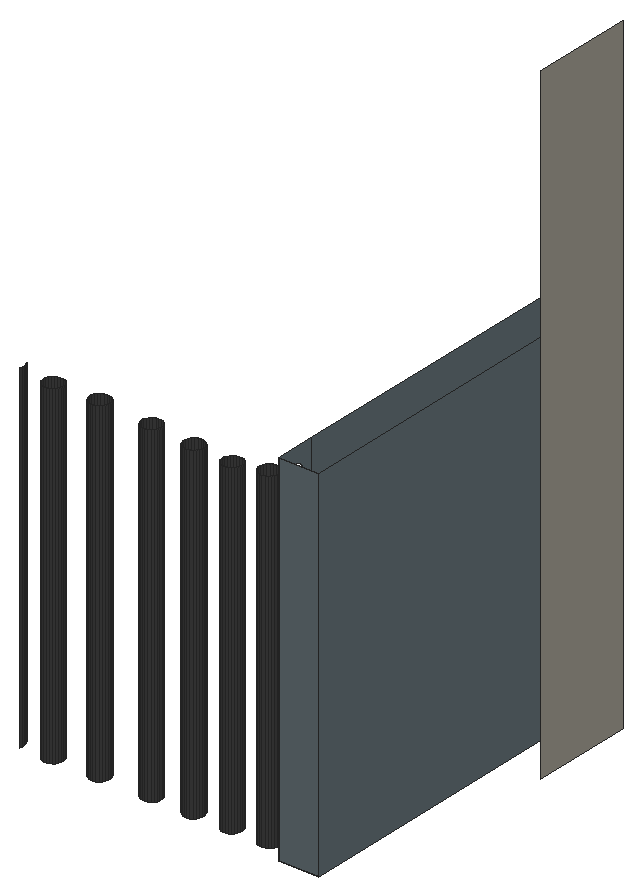
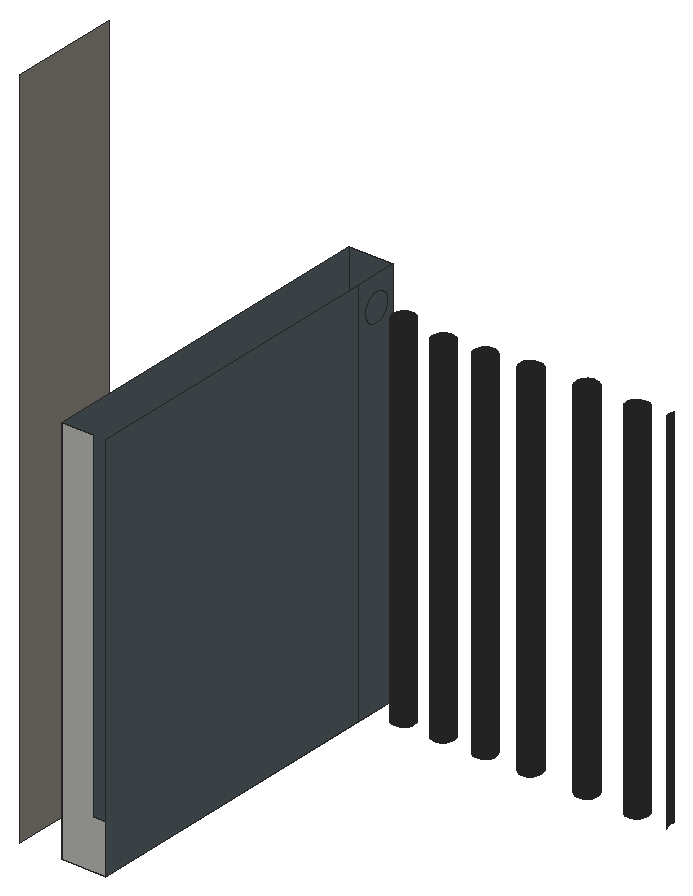
# SketchUp Ruby script. Lengths in inches.
U = 1.inch
M = Sketchup.active_model
def pt(a) = Geom::Point3d.new(a.map { |v| v * U })
def face(e, loops, mat)
  f = e.add_face(loops[0].map { |a| pt(a) })
  loops[1..].each { |l| e.add_face(l.map { |a| pt(a) }).erase! }
  f.material = f.back_material = mat if mat
  f
end
# faces: each face lists its corners as indices into pts; further lists are holes
def faces(e, pts, list, mat = nil) = list.each { |f| face(e, (f[0].is_a?(Array) ? f : [f]).map { |l| l.map { |i| pts[i] } }, mat) }
# xy, xz, yz: faces in a plane at the given z, y or x. An outline is a flat list of corners, or four numbers for a rectangle; further outlines are holes
def ring(l) = l.size == 4 ? [[l[0], l[1]], [l[2], l[1]], [l[2], l[3]], [l[0], l[3]]] : l.each_slice(2).to_a
def flat(e, list, mat, &to3) = list.each { |f| face(e, (f[0].is_a?(Array) ? f : [f]).map { |l| ring(l).map { |u, v| to3.(u, v) } }, mat) }
def xy(e, z, list, mat = nil) = flat(e, list, mat) { |x, y| [x, y, z] }
def xz(e, y, list, mat = nil) = flat(e, list, mat) { |x, z| [x, y, z] }
def yz(e, x, list, mat = nil) = flat(e, list, mat) { |y, z| [x, y, z] }
def lines(e, pts, list) = list.each { |a, b| e.add_line(pt(pts[a]), pt(pts[b])) }
# prism: a flat outline (further loops are holes) pulled along v
def prism(e, loops, v, mat = nil)
  f = face(e, loops, mat); d = Geom::Vector3d.new(v.map { |x| x * U })
  f.pushpull(f.normal.samedirection?(d) ? d.length : -d.length)
end
def box(e, o, s, mat = nil) = prism(e, [[o, [o[0] + s[0], o[1], o[2]], [o[0] + s[0], o[1] + s[1], o[2]], [o[0], o[1] + s[1], o[2]]]], [0, 0, s[2]], mat)
def at(x, y, z, deg = 0) = Geom::Transformation.translation(pt([x, y, z])) * Geom::Transformation.rotation(ORIGIN, Z_AXIS, deg.degrees)
def axes(o, x, y, z) = Geom::Transformation.new([*x, 0, *y, 0, *z, 0, *pt(o).to_a, 1])
def part(name) = M.definitions.add(name)
# library, detail: a bought-in or finely detailed component or shape, given as its bounding box
def library(name, o, s) = part(name).tap { |d| box(d.entities, o, s) }
def detail(e, o, s) = box(e.add_group.entities, o, s)
def put(e, d, t, mat = nil) = e.add_instance(d, t).tap { |i| i.material = mat if mat }
def group(e, t, mat = nil) = e.add_group.tap { |g| g.transformation = t; g.material = mat if mat }.entities
root = M.entities
M.materials.add("[Color M07]").color = [58, 58, 58]
M.materials.add("[Formica Graystone]").color = [149, 146, 135]
M.materials.add("[Formica Speckled Grey]").color = [94, 105, 111]
xy(root,334.79,[[295.92,120.91,298.73,144.04],[279.04,121.51,278.87,121.56,278.71,121.65,278.59,121.78,278.5,121.93,278.46,122.11,278.46,122.28,278.51,122.46,278.6,122.61,278.73,122.74,278.88,122.83,279.06,122.87,279.23,122.87,279.41,122.82,279.5625,122.73,279.6875,122.6,279.78,122.45,279.82,122.27,279.82,122.09,279.77,121.92,279.68,121.76,279.55,121.64,279.4,121.55,279.22,121.51],[282.29,121.51,282.12,121.56,281.96,121.65,281.84,121.78,281.75,121.93,281.71,122.11,281.71,122.28,281.76,122.46,281.85,122.61,281.98,122.74,282.13,122.83,282.31,122.87,282.48,122.87,282.66,122.82,282.8125,122.73,282.9375,122.6,283.03,122.45,283.07,122.27,283.07,122.09,283.02,121.92,282.93,121.76,282.8,121.64,282.65,121.55,282.47,121.51],[285.92,121.51,285.74,121.56,285.59,121.65,285.46,121.78,285.375,121.93,285.33,122.11,285.33,122.28,285.38,122.46,285.47,122.61,285.6,122.74,285.76,122.83,285.93,122.87,286.11,122.87,286.28,122.82,286.4375,122.73,286.5625,122.6,286.65,122.45,286.7,122.27,286.69,122.09,286.65,121.92,286.55,121.76,286.43,121.64,286.27,121.55,286.1,121.51],[288.85,121.51,288.68,121.56,288.53,121.65,288.4,121.78,288.3125,121.93,288.27,122.11,288.27,122.28,288.32,122.46,288.41,122.61,288.54,122.74,288.69,122.83,288.87,122.87,289.05,122.87,289.22,122.82,289.375,122.73,289.5,122.6,289.59,122.45,289.63,122.27,289.63,122.09,289.58,121.92,289.49,121.76,289.36,121.64,289.21,121.55,289.03,121.51],
  [291.54,121.51,291.37,121.56,291.21,121.65,291.09,121.78,291,121.93,290.96,122.11,290.96,122.28,291.01,122.46,291.1,122.61,291.23,122.74,291.38,122.83,291.56,122.87,291.73,122.87,291.91,122.82,292.0625,122.73,292.1875,122.6,292.28,122.45,292.32,122.27,292.32,122.09,292.27,121.92,292.18,121.76,292.05,121.64,291.9,121.55,291.72,121.51],[294.1,121.51,293.93,121.56,293.78,121.65,293.65,121.78,293.5625,121.93,293.52,122.11,293.52,122.28,293.57,122.46,293.66,122.61,293.79,122.74,293.94,122.83,294.12,122.87,294.3,122.87,294.47,122.82,294.625,122.73,294.75,122.6,294.84,122.45,294.88,122.27,294.88,122.09,294.83,121.92,294.74,121.76,294.61,121.64,294.46,121.55,294.28,121.51]])
xz(root,120.91,[[295.92,334.79,298.73,359.98]],"[Formica Speckled Grey]")
xz(root,121.51,[[279.04,334.79,279.22,358.23],[282.29,334.79,282.47,358.31],[285.92,334.79,286.1,358.07],[288.85,334.79,289.03,357.82],[291.54,334.79,291.72,357.67],
  [294.1,334.79,294.28,358.04]],"[Color M07]")
xz(root,122.87,[[279.06,334.79,279.23,358.23],[282.31,334.79,282.48,358.31],[285.93,334.79,286.11,358.07],[288.87,334.79,289.05,357.82],[291.56,334.79,291.73,357.67],
  [294.12,334.79,294.3,358.04]],"[Color M07]")
xz(root,144.04,[[295.92,334.79,298.73,334.79,298.73,359.98,296.73,359.98,296.73,337.93,295.92,337.93]])
yz(root,277.07,[[122.09,334.79,122.27,358.53]],"[Color M07]")
yz(root,278.46,[[122.11,334.79,122.28,358.23]],"[Color M07]")
yz(root,279.82,[[122.09,334.79,122.27,358.23]],"[Color M07]")
yz(root,281.71,[[122.11,334.79,122.28,358.31]],"[Color M07]")
yz(root,283.07,[[122.09,334.79,122.27,358.31]],"[Color M07]")
yz(root,285.33,[[122.11,334.79,122.28,358.07]],"[Color M07]")
yz(root,288.27,[[122.11,334.79,122.28,357.82]],"[Color M07]")
yz(root,289.63,[[122.09,334.79,122.27,357.82]],"[Color M07]")
yz(root,290.96,[[122.11,334.79,122.28,357.67]],"[Color M07]")
yz(root,292.32,[[122.09,334.79,122.27,357.67]],"[Color M07]")
yz(root,293.52,[[122.11,334.79,122.28,358.04]],"[Color M07]")
yz(root,294.88,[[122.09,334.79,122.27,358.04]],"[Color M07]")
yz(root,295.92,[[[120.91,334.79,123.73,359.98],[122.22,357.13,122.46,357.16,122.6875,357.25,122.88,357.4,123.03,357.6,123.125,357.82,123.16,358.07,123.125,358.31,123.03,358.53,122.88,358.73,122.6875,358.88,122.46,358.97,122.22,359,121.97,358.97,121.75,358.88,121.55,358.73,121.41,358.53,121.3125,358.31,121.28,358.07,121.3125,357.82,121.41,357.6,121.55,357.4,121.75,357.25,121.97,357.16]],[123.73,334.79,144.04,359.98]],"[Formica Speckled Grey]")
yz(root,298.73,[[120.91,334.79,144.04,359.98]],"[Formica Speckled Grey]")
yz(root,301.43,[[136.91,334.79,144.04,379.13]],"[Formica Graystone]")
p = [[278.87,121.56,334.79],[279.04,121.51,334.79],[279.04,121.51,358.23],[278.87,121.56,358.23],[278.87,121.56,357.4],[279.22,121.51,334.79],
  [279.4,121.55,334.79],[279.4,121.55,358.23],[279.22,121.51,358.23],[282.12,121.56,334.79],[282.29,121.51,334.79],[282.29,121.51,358.31],
  [282.12,121.56,358.31],[282.12,121.56,357.4],[282.47,121.51,334.79],[282.65,121.55,334.79],[282.65,121.55,358.31],[282.47,121.51,358.31],
  [285.74,121.56,334.79],[285.92,121.51,334.79],[285.92,121.51,358.07],[285.74,121.56,358.07],[285.74,121.56,357.4],[286.1,121.51,334.79],
  [286.27,121.55,334.79],[286.27,121.55,358.07],[286.1,121.51,358.07],[288.68,121.56,334.79],[288.85,121.51,334.79],[288.85,121.51,357.82],
  [288.68,121.56,357.82],[288.68,121.56,357.4],[289.03,121.51,334.79],[289.21,121.55,334.79],[289.21,121.55,357.82],[289.03,121.51,357.82],
  [291.37,121.56,334.79],[291.54,121.51,334.79],[291.54,121.51,357.67],[291.37,121.56,357.67],[291.37,121.56,357.4],[291.72,121.51,334.79],
  [291.9,121.55,334.79],[291.9,121.55,357.67],[291.72,121.51,357.67],[293.93,121.56,334.79],[294.1,121.51,334.79],[294.1,121.51,358.04],
  [293.93,121.56,358.04],[293.93,121.56,357.4],[294.28,121.51,334.79],[294.46,121.55,334.79],[294.46,121.55,358.04],[294.28,121.51,358.04],
  [278.59,121.78,334.79],[278.71,121.65,334.79],[278.71,121.65,358.23],[278.59,121.78,358.23],[279.55,121.64,334.79],[279.55,121.64,358.23],
  [279.68,121.76,334.79],[279.68,121.76,358.23],[281.84,121.78,334.79],[281.96,121.65,334.79],[281.96,121.65,358.31],[281.84,121.78,358.31],
  [282.8,121.64,334.79],[282.8,121.64,358.31],[282.93,121.76,334.79],[282.93,121.76,358.31],[285.46,121.78,334.79],[285.59,121.65,334.79],
  [285.59,121.65,358.07],[285.46,121.78,358.07],[286.43,121.64,334.79],[286.43,121.64,358.07],[286.55,121.76,334.79],[286.55,121.76,358.07],
  [288.4,121.78,334.79],[288.53,121.65,334.79],[288.53,121.65,357.82],[288.4,121.78,357.82],[289.36,121.64,334.79],[289.36,121.64,357.82],
  [289.49,121.76,334.79],[289.49,121.76,357.82],[291.09,121.78,334.79],[291.21,121.65,334.79],[291.21,121.65,357.67],[291.09,121.78,357.67],
  [292.05,121.64,334.79],[292.05,121.64,357.67],[292.18,121.76,334.79],[292.18,121.76,357.67],[293.65,121.78,334.79],[293.78,121.65,334.79],
  [293.78,121.65,358.04],[293.65,121.78,358.04],[294.61,121.64,334.79],[294.61,121.64,358.04],[294.74,121.76,334.79],[294.74,121.76,358.04],
  [278.5,121.93,334.79],[278.5,121.93,358.23],[279.77,121.92,334.79],[279.77,121.92,358.23],[281.75,121.93,334.79],[281.75,121.93,358.31],
  [283.02,121.92,334.79],[283.02,121.92,358.31],[285.375,121.93,334.79],[285.375,121.93,358.07],[286.65,121.92,334.79],[286.65,121.92,358.07],
  [288.3125,121.93,334.79],[288.3125,121.93,357.82],[289.58,121.92,334.79],[289.58,121.92,357.82],[291,121.93,334.79],[291,121.93,357.67],
  [292.27,121.92,334.79],[292.27,121.92,357.67],[293.5625,121.93,334.79],[293.5625,121.93,358.04],[294.83,121.92,334.79],[294.83,121.92,358.04],
  [277.02,121.92,334.79],[277.07,122.09,334.79],[277.07,122.09,358.53],[277.02,121.92,358.53],[278.46,122.11,334.79],[278.46,122.11,358.23],
  [279.82,122.09,334.79],[279.82,122.09,358.23],[281.71,122.11,334.79],[281.71,122.11,358.31],[283.07,122.09,334.79],[283.07,122.09,358.31],
  [285.33,122.11,334.79],[285.33,122.11,358.07],[286.69,122.09,334.79],[286.69,122.09,358.07],[288.27,122.11,334.79],[288.27,122.11,357.82],
  [289.63,122.09,334.79],[289.63,122.09,357.82],[290.96,122.11,334.79],[290.96,122.11,357.67],[292.32,122.09,334.79],[292.32,122.09,357.67],
  [293.52,122.11,334.79],[293.52,122.11,358.04],[294.88,122.09,334.79],[294.88,122.09,358.04],[286.7,122.27,334.79],[286.7,122.27,358.07],
  [277.07,122.27,334.79],[277.03,122.45,334.79],[277.03,122.45,358.53],[277.07,122.27,358.53],[278.51,122.46,334.79],[278.46,122.28,334.79],
  [278.46,122.28,358.23],[278.51,122.46,358.23],[279.82,122.27,334.79],[279.78,122.45,334.79],[279.78,122.45,358.23],[279.82,122.27,358.23],
  [281.76,122.46,334.79],[281.71,122.28,334.79],[281.71,122.28,358.31],[281.76,122.46,358.31],[283.07,122.27,334.79],[283.03,122.45,334.79],
  [283.03,122.45,358.31],[283.07,122.27,358.31],[285.38,122.46,334.79],[285.33,122.28,334.79],[285.33,122.28,358.07],[285.38,122.46,358.07],
  [286.65,122.45,334.79],[286.65,122.45,358.07],[288.32,122.46,334.79],[288.27,122.28,334.79],[288.27,122.28,357.82],[288.32,122.46,357.82],
  [289.63,122.27,334.79],[289.59,122.45,334.79],[289.59,122.45,357.82],[289.63,122.27,357.82],[291.01,122.46,334.79],[290.96,122.28,334.79],
  [290.96,122.28,357.67],[291.01,122.46,357.67],[292.32,122.27,334.79],[292.28,122.45,334.79],[292.28,122.45,357.67],[292.32,122.27,357.67],
  [293.57,122.46,334.79],[293.52,122.28,334.79],[293.52,122.28,358.04],[293.57,122.46,358.04],[294.88,122.27,334.79],[294.84,122.45,334.79],
  [294.84,122.45,358.04],[294.88,122.27,358.04],[276.9375,122.6,334.79],[276.9375,122.6,358.53],[279.6875,122.6,334.79],[279.6875,122.6,358.23],
  [282.9375,122.6,334.79],[282.9375,122.6,358.31],[286.5625,122.6,334.79],[286.5625,122.6,358.07],[289.5,122.6,334.79],[289.5,122.6,357.82],
  [292.1875,122.6,334.79],[292.1875,122.6,357.67],[294.75,122.6,334.79],[294.75,122.6,358.04],[278.6,122.61,334.79],[278.6,122.61,358.23],
  [281.85,122.61,334.79],[281.85,122.61,358.31],[285.47,122.61,334.79],[285.47,122.61,358.07],[288.41,122.61,334.79],[288.41,122.61,357.82],
  [291.1,122.61,334.79],[291.1,122.61,357.67],[293.66,122.61,334.79],[293.66,122.61,358.04],[278.73,122.74,334.79],[278.73,122.74,358.23],
  [279.5625,122.73,334.79],[279.5625,122.73,358.23],[281.98,122.74,334.79],[281.98,122.74,358.31],[282.8125,122.73,334.79],[282.8125,122.73,358.31],
  [285.6,122.74,334.79],[285.6,122.74,358.07],[286.4375,122.73,334.79],[286.4375,122.73,358.07],[288.54,122.74,334.79],[288.54,122.74,357.82],
  [289.375,122.73,334.79],[289.375,122.73,357.82],[291.23,122.74,334.79],[291.23,122.74,357.67],[292.0625,122.73,334.79],[292.0625,122.73,357.67],
  [293.79,122.74,334.79],[293.79,122.74,358.04],[294.625,122.73,334.79],[294.625,122.73,358.04],[278.88,122.83,334.79],[278.88,122.83,358.23],
  [279.41,122.82,334.79],[279.41,122.82,358.23],[282.13,122.83,334.79],[282.13,122.83,358.31],[282.66,122.82,334.79],[282.66,122.82,358.31],
  [285.76,122.83,334.79],[285.76,122.83,358.07],[286.28,122.82,334.79],[286.28,122.82,358.07],[288.69,122.83,334.79],[288.69,122.83,357.82],
  [289.22,122.82,334.79],[289.22,122.82,357.82],[291.38,122.83,334.79],[291.38,122.83,357.67],[291.91,122.82,334.79],[291.91,122.82,357.67],
  [293.94,122.83,334.79],[293.94,122.83,358.04],[294.47,122.82,334.79],[294.47,122.82,358.04],[279.06,122.87,334.79],[279.06,122.87,358.23],
  [279.23,122.87,334.79],[279.23,122.87,358.23],[282.31,122.87,334.79],[282.31,122.87,358.31],[282.48,122.87,334.79],[282.48,122.87,358.31],
  [285.93,122.87,334.79],[285.93,122.87,358.07],[286.11,122.87,334.79],[286.11,122.87,358.07],[288.87,122.87,334.79],[288.87,122.87,357.82],
  [289.05,122.87,334.79],[289.05,122.87,357.82],[291.56,122.87,334.79],[291.56,122.87,357.67],[291.73,122.87,334.79],[291.73,122.87,357.67],
  [294.12,122.87,334.79],[294.12,122.87,358.04],[294.3,122.87,334.79],[294.3,122.87,358.04]]
faces(root,p,[[0,1,2,3,4],[5,6,7,8],[9,10,11,12,13],[14,15,16,17],[18,19,20,21,22],[23,24,25,26],[27,28,29,30,31],[32,33,34,35],
  [36,37,38,39,40],[41,42,43,44],[45,46,47,48,49],[50,51,52,53],[54,55,56,57],[55,0,4,3,56],[6,58,59,7],[58,60,61,59],
  [62,63,64,65],[63,9,13,12,64],[15,66,67,16],[66,68,69,67],[70,71,72,73],[71,18,22,21,72],[24,74,75,25],[74,76,77,75],
  [78,79,80,81],[79,27,31,30,80],[33,82,83,34],[82,84,85,83],[86,87,88,89],[87,36,40,39,88],[42,90,91,43],[90,92,93,91],
  [94,95,96,97],[95,45,49,48,96],[51,98,99,52],[98,100,101,99],[102,54,57,103],[60,104,105,61],[106,62,65,107],[68,108,109,69],
  [110,70,73,111],[76,112,113,77],[114,78,81,115],[84,116,117,85],[118,86,89,119],[92,120,121,93],[122,94,97,123],[100,124,125,101],
  [126,127,128,129],[130,102,103,131],[104,132,133,105],[134,106,107,135],[108,136,137,109],[138,110,111,139],[112,140,141,113],[142,114,115,143],
  [116,144,145,117],[146,118,119,147],[120,148,149,121],[150,122,123,151],[124,152,153,125],[140,154,155,141],[156,157,158,159],[160,161,162,163],
  [164,165,166,167],[168,169,170,171],[172,173,174,175],[176,177,178,179],[154,180,181,155],[182,183,184,185],[186,187,188,189],[190,191,192,193],
  [194,195,196,197],[198,199,200,201],[202,203,204,205],[157,206,207,158],[165,208,209,166],[173,210,211,174],[180,212,213,181],[187,214,215,188],
  [195,216,217,196],[203,218,219,204],[220,160,163,221],[222,168,171,223],[224,176,179,225],[226,182,185,227],[228,190,193,229],[230,198,201,231],
  [232,220,221,233],[208,234,235,209],[236,222,223,237],[210,238,239,211],[240,224,225,241],[212,242,243,213],[244,226,227,245],[214,246,247,215],
  [248,228,229,249],[216,250,251,217],[252,230,231,253],[218,254,255,219],[256,232,233,257],[234,258,259,235],[260,236,237,261],[238,262,263,239],
  [264,240,241,265],[242,266,267,243],[268,244,245,269],[246,270,271,247],[272,248,249,273],[250,274,275,251],[276,252,253,277],[254,278,279,255],
  [280,256,257,281],[258,282,283,259],[284,260,261,285],[262,286,287,263],[288,264,265,289],[266,290,291,267],[292,268,269,293],[270,294,295,271],
  [296,272,273,297],[274,298,299,275],[300,276,277,301],[278,302,303,279]],"[Color M07]")
